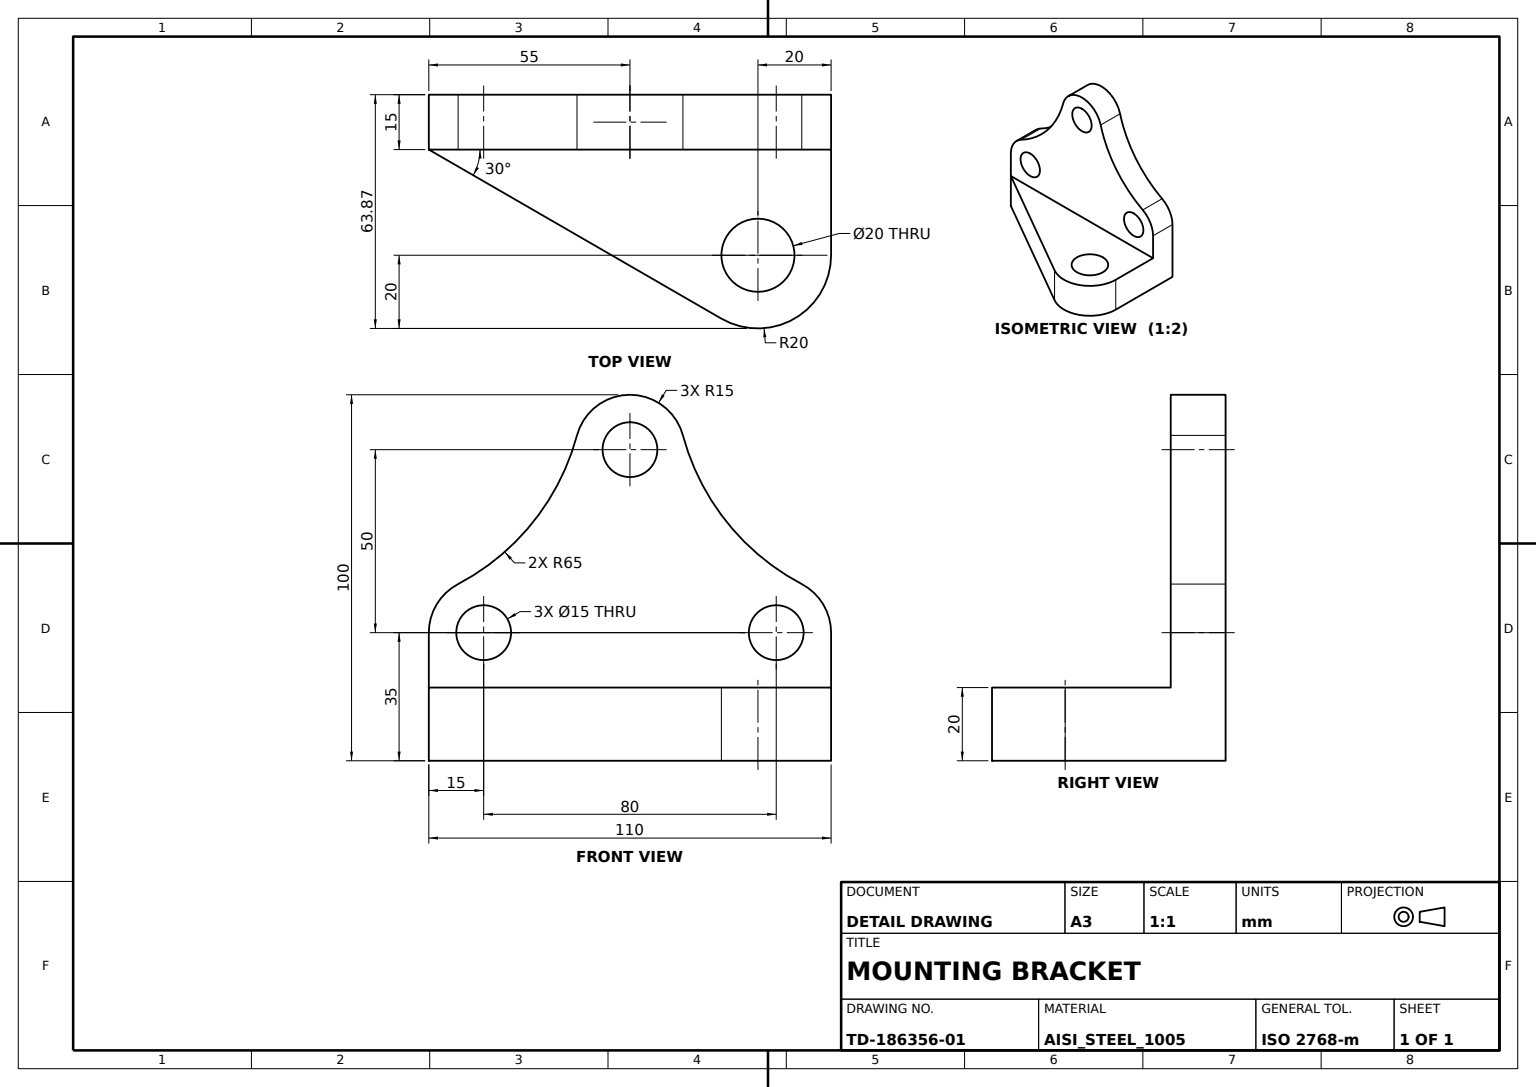
ISO-10303-21;
HEADER;
FILE_DESCRIPTION((''),'2;1');
FILE_NAME('','',(''),(''),'','','');
FILE_SCHEMA(('AUTOMOTIVE_DESIGN'));
ENDSEC;
DATA;
#1=APPLICATION_CONTEXT('');
#2=PRODUCT_CONTEXT('',#1,'mechanical');
#3=PRODUCT('','','',(#2));
#4=PRODUCT_DEFINITION_FORMATION('','',#3);
#5=PRODUCT_DEFINITION_CONTEXT('',#1,'design');
#6=PRODUCT_DEFINITION('','',#4,#5);
#7=PRODUCT_DEFINITION_SHAPE('','',#6);
#8=(LENGTH_UNIT()NAMED_UNIT(*)SI_UNIT(.MILLI.,.METRE.));
#9=(NAMED_UNIT(*)PLANE_ANGLE_UNIT()SI_UNIT($,.RADIAN.));
#10=(NAMED_UNIT(*)SI_UNIT($,.STERADIAN.)SOLID_ANGLE_UNIT());
#11=UNCERTAINTY_MEASURE_WITH_UNIT(LENGTH_MEASURE(0.005),#8,'distance_accuracy_value','');
#12=(GEOMETRIC_REPRESENTATION_CONTEXT(3)GLOBAL_UNCERTAINTY_ASSIGNED_CONTEXT((#11))GLOBAL_UNIT_ASSIGNED_CONTEXT((#8,#9,#10))REPRESENTATION_CONTEXT('',''));
#13=CARTESIAN_POINT('',(20.,0.,92.5));
#14=VERTEX_POINT('',#13);
#15=CARTESIAN_POINT('',(20.,0.,85.));
#16=DIRECTION('',(-1.,0.,0.));
#17=DIRECTION('',(0.,0.,1.));
#18=AXIS2_PLACEMENT_3D('',#15,#16,#17);
#19=CIRCLE('',#18,7.5);
#20=EDGE_CURVE('',#14,#14,#19,.T.);
#21=ORIENTED_EDGE('',*,*,#20,.T.);
#22=EDGE_LOOP('',(#21));
#23=FACE_BOUND('',#22,.T.);
#24=CARTESIAN_POINT('',(20.,40.,42.5));
#25=VERTEX_POINT('',#24);
#26=CARTESIAN_POINT('',(20.,40.,35.));
#27=AXIS2_PLACEMENT_3D('',#26,#16,#17);
#28=CIRCLE('',#27,7.5);
#29=EDGE_CURVE('',#25,#25,#28,.T.);
#30=ORIENTED_EDGE('',*,*,#29,.T.);
#31=EDGE_LOOP('',(#30));
#32=FACE_BOUND('',#31,.T.);
#33=CARTESIAN_POINT('',(20.,55.,20.));
#34=VERTEX_POINT('',#33);
#35=CARTESIAN_POINT('',(20.,55.,35.));
#36=VERTEX_POINT('',#35);
#37=CARTESIAN_POINT('',(20.,55.,0.));
#38=VECTOR('',#17,1000.);
#39=LINE('',#37,#38);
#40=EDGE_CURVE('',#34,#36,#39,.T.);
#41=ORIENTED_EDGE('',*,*,#40,.T.);
#42=CARTESIAN_POINT('',(20.,46.984173,48.274838));
#43=VERTEX_POINT('',#42);
#44=DIRECTION('',(1.,0.,0.));
#45=DIRECTION('',(0.,1.,0.));
#46=AXIS2_PLACEMENT_3D('',#26,#44,#45);
#47=CIRCLE('',#46,15.);
#48=EDGE_CURVE('',#36,#43,#47,.T.);
#49=ORIENTED_EDGE('',*,*,#48,.T.);
#50=CARTESIAN_POINT('',(20.,14.484173,88.899838));
#51=VERTEX_POINT('',#50);
#52=CARTESIAN_POINT('',(20.,77.248922,105.799137));
#53=DIRECTION('',(0.,-1.,0.));
#54=AXIS2_PLACEMENT_3D('',#52,#16,#53);
#55=CIRCLE('',#54,65.);
#56=EDGE_CURVE('',#43,#51,#55,.T.);
#57=ORIENTED_EDGE('',*,*,#56,.T.);
#58=CARTESIAN_POINT('',(20.,-14.484173,88.899838));
#59=VERTEX_POINT('',#58);
#60=AXIS2_PLACEMENT_3D('',#15,#44,#45);
#61=CIRCLE('',#60,15.);
#62=EDGE_CURVE('',#51,#59,#61,.T.);
#63=ORIENTED_EDGE('',*,*,#62,.T.);
#64=CARTESIAN_POINT('',(20.,-46.984173,48.274838));
#65=VERTEX_POINT('',#64);
#66=CARTESIAN_POINT('',(20.,-77.248922,105.799137));
#67=AXIS2_PLACEMENT_3D('',#66,#16,#45);
#68=CIRCLE('',#67,65.);
#69=EDGE_CURVE('',#59,#65,#68,.T.);
#70=ORIENTED_EDGE('',*,*,#69,.T.);
#71=CARTESIAN_POINT('',(20.,-55.,35.));
#72=VERTEX_POINT('',#71);
#73=CARTESIAN_POINT('',(20.,-40.,35.));
#74=AXIS2_PLACEMENT_3D('',#73,#44,#45);
#75=CIRCLE('',#74,15.);
#76=EDGE_CURVE('',#65,#72,#75,.T.);
#77=ORIENTED_EDGE('',*,*,#76,.T.);
#78=CARTESIAN_POINT('',(20.,-55.,20.));
#79=VERTEX_POINT('',#78);
#80=DIRECTION('',(0.,0.,-1.));
#81=VECTOR('',#80,1000.);
#82=LINE('',#71,#81);
#83=EDGE_CURVE('',#72,#79,#82,.T.);
#84=ORIENTED_EDGE('',*,*,#83,.T.);
#85=VECTOR('',#53,1000.);
#86=LINE('',#33,#85);
#87=EDGE_CURVE('',#34,#79,#86,.T.);
#88=ORIENTED_EDGE('',*,*,#87,.F.);
#89=EDGE_LOOP('',(#41,#49,#57,#63,#70,#77,#84,#88));
#90=FACE_BOUND('',#89,.T.);
#91=CARTESIAN_POINT('',(20.,-40.,42.5));
#92=VERTEX_POINT('',#91);
#93=AXIS2_PLACEMENT_3D('',#73,#16,#17);
#94=CIRCLE('',#93,7.5);
#95=EDGE_CURVE('',#92,#92,#94,.T.);
#96=ORIENTED_EDGE('',*,*,#95,.T.);
#97=EDGE_LOOP('',(#96));
#98=FACE_BOUND('',#97,.T.);
#99=AXIS2_PLACEMENT_3D('',#26,#44,#80);
#100=PLANE('',#99);
#101=ADVANCED_FACE('',(#23,#32,#90,#98),#100,.T.);
#102=ORIENTED_EDGE('',*,*,#95,.F.);
#103=EDGE_LOOP('',(#102));
#104=FACE_BOUND('',#103,.T.);
#105=CARTESIAN_POINT('',(5.,-40.,27.5));
#106=VERTEX_POINT('',#105);
#107=CARTESIAN_POINT('',(5.,-40.,35.));
#108=AXIS2_PLACEMENT_3D('',#107,#44,#80);
#109=CIRCLE('',#108,7.5);
#110=EDGE_CURVE('',#106,#106,#109,.T.);
#111=ORIENTED_EDGE('',*,*,#110,.F.);
#112=EDGE_LOOP('',(#111));
#113=FACE_BOUND('',#112,.T.);
#114=CYLINDRICAL_SURFACE('',#93,7.5);
#115=ADVANCED_FACE('',(#104,#113),#114,.F.);
#116=CARTESIAN_POINT('',(5.,40.,27.5));
#117=VERTEX_POINT('',#116);
#118=CARTESIAN_POINT('',(5.,40.,35.));
#119=AXIS2_PLACEMENT_3D('',#118,#44,#80);
#120=CIRCLE('',#119,7.5);
#121=EDGE_CURVE('',#117,#117,#120,.T.);
#122=ORIENTED_EDGE('',*,*,#121,.F.);
#123=EDGE_LOOP('',(#122));
#124=FACE_BOUND('',#123,.T.);
#125=ORIENTED_EDGE('',*,*,#29,.F.);
#126=EDGE_LOOP('',(#125));
#127=FACE_BOUND('',#126,.T.);
#128=CYLINDRICAL_SURFACE('',#27,7.5);
#129=ADVANCED_FACE('',(#124,#127),#128,.F.);
#130=CARTESIAN_POINT('',(66.188022,25.,20.));
#131=VERTEX_POINT('',#130);
#132=DIRECTION('',(0.5,0.866025404,0.));
#133=VECTOR('',#132,1000.);
#134=LINE('',#78,#133);
#135=EDGE_CURVE('',#79,#131,#134,.T.);
#136=ORIENTED_EDGE('',*,*,#135,.F.);
#137=CARTESIAN_POINT('',(20.,-55.,0.));
#138=VERTEX_POINT('',#137);
#139=LINE('',#78,#81);
#140=EDGE_CURVE('',#79,#138,#139,.T.);
#141=ORIENTED_EDGE('',*,*,#140,.T.);
#142=CARTESIAN_POINT('',(66.188022,25.,0.));
#143=VERTEX_POINT('',#142);
#144=LINE('',#137,#133);
#145=EDGE_CURVE('',#138,#143,#144,.T.);
#146=ORIENTED_EDGE('',*,*,#145,.T.);
#147=LINE('',#130,#81);
#148=EDGE_CURVE('',#131,#143,#147,.T.);
#149=ORIENTED_EDGE('',*,*,#148,.F.);
#150=EDGE_LOOP('',(#136,#141,#146,#149));
#151=FACE_BOUND('',#150,.T.);
#152=DIRECTION('',(-0.866025404,0.5,0.));
#153=DIRECTION('',(-0.5,-0.866025404,0.));
#154=AXIS2_PLACEMENT_3D('',#78,#152,#153);
#155=PLANE('',#154);
#156=ADVANCED_FACE('',(#151),#155,.F.);
#157=ORIENTED_EDGE('',*,*,#20,.F.);
#158=EDGE_LOOP('',(#157));
#159=FACE_BOUND('',#158,.T.);
#160=CARTESIAN_POINT('',(5.,0.,77.5));
#161=VERTEX_POINT('',#160);
#162=CARTESIAN_POINT('',(5.,0.,85.));
#163=AXIS2_PLACEMENT_3D('',#162,#44,#80);
#164=CIRCLE('',#163,7.5);
#165=EDGE_CURVE('',#161,#161,#164,.T.);
#166=ORIENTED_EDGE('',*,*,#165,.F.);
#167=EDGE_LOOP('',(#166));
#168=FACE_BOUND('',#167,.T.);
#169=CYLINDRICAL_SURFACE('',#18,7.5);
#170=ADVANCED_FACE('',(#159,#168),#169,.F.);
#171=ORIENTED_EDGE('',*,*,#165,.T.);
#172=EDGE_LOOP('',(#171));
#173=FACE_BOUND('',#172,.T.);
#174=CARTESIAN_POINT('',(5.,-55.,35.));
#175=VERTEX_POINT('',#174);
#176=CARTESIAN_POINT('',(5.,-55.,0.));
#177=VERTEX_POINT('',#176);
#178=LINE('',#174,#81);
#179=EDGE_CURVE('',#175,#177,#178,.T.);
#180=ORIENTED_EDGE('',*,*,#179,.F.);
#181=CARTESIAN_POINT('',(5.,-46.984173,48.274838));
#182=VERTEX_POINT('',#181);
#183=AXIS2_PLACEMENT_3D('',#107,#44,#45);
#184=CIRCLE('',#183,15.);
#185=EDGE_CURVE('',#182,#175,#184,.T.);
#186=ORIENTED_EDGE('',*,*,#185,.F.);
#187=CARTESIAN_POINT('',(5.,-14.484173,88.899838));
#188=VERTEX_POINT('',#187);
#189=CARTESIAN_POINT('',(5.,-77.248922,105.799137));
#190=AXIS2_PLACEMENT_3D('',#189,#16,#45);
#191=CIRCLE('',#190,65.);
#192=EDGE_CURVE('',#188,#182,#191,.T.);
#193=ORIENTED_EDGE('',*,*,#192,.F.);
#194=CARTESIAN_POINT('',(5.,14.484173,88.899838));
#195=VERTEX_POINT('',#194);
#196=AXIS2_PLACEMENT_3D('',#162,#44,#45);
#197=CIRCLE('',#196,15.);
#198=EDGE_CURVE('',#195,#188,#197,.T.);
#199=ORIENTED_EDGE('',*,*,#198,.F.);
#200=CARTESIAN_POINT('',(5.,46.984173,48.274838));
#201=VERTEX_POINT('',#200);
#202=CARTESIAN_POINT('',(5.,77.248922,105.799137));
#203=AXIS2_PLACEMENT_3D('',#202,#16,#53);
#204=CIRCLE('',#203,65.);
#205=EDGE_CURVE('',#201,#195,#204,.T.);
#206=ORIENTED_EDGE('',*,*,#205,.F.);
#207=CARTESIAN_POINT('',(5.,55.,35.));
#208=VERTEX_POINT('',#207);
#209=AXIS2_PLACEMENT_3D('',#118,#44,#45);
#210=CIRCLE('',#209,15.);
#211=EDGE_CURVE('',#208,#201,#210,.T.);
#212=ORIENTED_EDGE('',*,*,#211,.F.);
#213=CARTESIAN_POINT('',(5.,55.,0.));
#214=VERTEX_POINT('',#213);
#215=LINE('',#213,#38);
#216=EDGE_CURVE('',#214,#208,#215,.T.);
#217=ORIENTED_EDGE('',*,*,#216,.F.);
#218=VECTOR('',#45,1000.);
#219=LINE('',#176,#218);
#220=EDGE_CURVE('',#177,#214,#219,.T.);
#221=ORIENTED_EDGE('',*,*,#220,.F.);
#222=EDGE_LOOP('',(#180,#186,#193,#199,#206,#212,#217,#221));
#223=FACE_BOUND('',#222,.T.);
#224=ORIENTED_EDGE('',*,*,#121,.T.);
#225=EDGE_LOOP('',(#224));
#226=FACE_BOUND('',#225,.T.);
#227=ORIENTED_EDGE('',*,*,#110,.T.);
#228=EDGE_LOOP('',(#227));
#229=FACE_BOUND('',#228,.T.);
#230=PLANE('',#119);
#231=ADVANCED_FACE('',(#173,#223,#226,#229),#230,.F.);
#232=VECTOR('',#16,1000.);
#233=LINE('',#137,#232);
#234=EDGE_CURVE('',#138,#177,#233,.T.);
#235=ORIENTED_EDGE('',*,*,#234,.F.);
#236=ORIENTED_EDGE('',*,*,#140,.F.);
#237=ORIENTED_EDGE('',*,*,#83,.F.);
#238=LINE('',#71,#232);
#239=EDGE_CURVE('',#72,#175,#238,.T.);
#240=ORIENTED_EDGE('',*,*,#239,.T.);
#241=ORIENTED_EDGE('',*,*,#179,.T.);
#242=EDGE_LOOP('',(#235,#236,#237,#240,#241));
#243=FACE_BOUND('',#242,.T.);
#244=AXIS2_PLACEMENT_3D('',#71,#45,#17);
#245=PLANE('',#244);
#246=ADVANCED_FACE('',(#243),#245,.F.);
#247=ORIENTED_EDGE('',*,*,#62,.F.);
#248=LINE('',#50,#232);
#249=EDGE_CURVE('',#51,#195,#248,.T.);
#250=ORIENTED_EDGE('',*,*,#249,.T.);
#251=ORIENTED_EDGE('',*,*,#198,.T.);
#252=LINE('',#58,#232);
#253=EDGE_CURVE('',#59,#188,#252,.T.);
#254=ORIENTED_EDGE('',*,*,#253,.F.);
#255=EDGE_LOOP('',(#247,#250,#251,#254));
#256=FACE_BOUND('',#255,.T.);
#257=CYLINDRICAL_SURFACE('',#18,15.);
#258=ADVANCED_FACE('',(#256),#257,.T.);
#259=ORIENTED_EDGE('',*,*,#249,.F.);
#260=ORIENTED_EDGE('',*,*,#56,.F.);
#261=LINE('',#42,#232);
#262=EDGE_CURVE('',#43,#201,#261,.T.);
#263=ORIENTED_EDGE('',*,*,#262,.T.);
#264=ORIENTED_EDGE('',*,*,#205,.T.);
#265=EDGE_LOOP('',(#259,#260,#263,#264));
#266=FACE_BOUND('',#265,.T.);
#267=AXIS2_PLACEMENT_3D('',#52,#16,#17);
#268=CYLINDRICAL_SURFACE('',#267,65.);
#269=ADVANCED_FACE('',(#266),#268,.F.);
#270=CARTESIAN_POINT('',(38.867513,35.,20.));
#271=VERTEX_POINT('',#270);
#272=CARTESIAN_POINT('',(48.867513,35.,20.));
#273=AXIS2_PLACEMENT_3D('',#272,#80,#16);
#274=CIRCLE('',#273,10.);
#275=EDGE_CURVE('',#271,#271,#274,.T.);
#276=ORIENTED_EDGE('',*,*,#275,.F.);
#277=EDGE_LOOP('',(#276));
#278=FACE_BOUND('',#277,.T.);
#279=CARTESIAN_POINT('',(58.867513,35.,0.));
#280=VERTEX_POINT('',#279);
#281=CARTESIAN_POINT('',(48.867513,35.,0.));
#282=AXIS2_PLACEMENT_3D('',#281,#17,#44);
#283=CIRCLE('',#282,10.);
#284=EDGE_CURVE('',#280,#280,#283,.T.);
#285=ORIENTED_EDGE('',*,*,#284,.F.);
#286=EDGE_LOOP('',(#285));
#287=FACE_BOUND('',#286,.T.);
#288=CYLINDRICAL_SURFACE('',#273,10.);
#289=ADVANCED_FACE('',(#278,#287),#288,.F.);
#290=ORIENTED_EDGE('',*,*,#148,.T.);
#291=CARTESIAN_POINT('',(48.867513,55.,0.));
#292=VERTEX_POINT('',#291);
#293=CIRCLE('',#282,20.);
#294=EDGE_CURVE('',#143,#292,#293,.T.);
#295=ORIENTED_EDGE('',*,*,#294,.T.);
#296=CARTESIAN_POINT('',(48.867513,55.,20.));
#297=VERTEX_POINT('',#296);
#298=LINE('',#296,#81);
#299=EDGE_CURVE('',#297,#292,#298,.T.);
#300=ORIENTED_EDGE('',*,*,#299,.F.);
#301=AXIS2_PLACEMENT_3D('',#272,#17,#44);
#302=CIRCLE('',#301,20.);
#303=EDGE_CURVE('',#131,#297,#302,.T.);
#304=ORIENTED_EDGE('',*,*,#303,.F.);
#305=EDGE_LOOP('',(#290,#295,#300,#304));
#306=FACE_BOUND('',#305,.T.);
#307=CYLINDRICAL_SURFACE('',#273,20.);
#308=ADVANCED_FACE('',(#306),#307,.T.);
#309=ORIENTED_EDGE('',*,*,#87,.T.);
#310=ORIENTED_EDGE('',*,*,#135,.T.);
#311=ORIENTED_EDGE('',*,*,#303,.T.);
#312=LINE('',#296,#232);
#313=EDGE_CURVE('',#297,#34,#312,.T.);
#314=ORIENTED_EDGE('',*,*,#313,.T.);
#315=EDGE_LOOP('',(#309,#310,#311,#314));
#316=FACE_BOUND('',#315,.T.);
#317=ORIENTED_EDGE('',*,*,#275,.T.);
#318=EDGE_LOOP('',(#317));
#319=FACE_BOUND('',#318,.T.);
#320=PLANE('',#301);
#321=ADVANCED_FACE('',(#316,#319),#320,.T.);
#322=LINE('',#35,#232);
#323=EDGE_CURVE('',#36,#208,#322,.T.);
#324=ORIENTED_EDGE('',*,*,#323,.T.);
#325=ORIENTED_EDGE('',*,*,#211,.T.);
#326=ORIENTED_EDGE('',*,*,#262,.F.);
#327=ORIENTED_EDGE('',*,*,#48,.F.);
#328=EDGE_LOOP('',(#324,#325,#326,#327));
#329=FACE_BOUND('',#328,.T.);
#330=CYLINDRICAL_SURFACE('',#27,15.);
#331=ADVANCED_FACE('',(#329),#330,.T.);
#332=ORIENTED_EDGE('',*,*,#299,.T.);
#333=LINE('',#291,#232);
#334=EDGE_CURVE('',#292,#214,#333,.T.);
#335=ORIENTED_EDGE('',*,*,#334,.T.);
#336=ORIENTED_EDGE('',*,*,#216,.T.);
#337=ORIENTED_EDGE('',*,*,#323,.F.);
#338=ORIENTED_EDGE('',*,*,#40,.F.);
#339=ORIENTED_EDGE('',*,*,#313,.F.);
#340=EDGE_LOOP('',(#332,#335,#336,#337,#338,#339));
#341=FACE_BOUND('',#340,.T.);
#342=AXIS2_PLACEMENT_3D('',#296,#53,#80);
#343=PLANE('',#342);
#344=ADVANCED_FACE('',(#341),#343,.F.);
#345=ORIENTED_EDGE('',*,*,#284,.T.);
#346=EDGE_LOOP('',(#345));
#347=FACE_BOUND('',#346,.T.);
#348=ORIENTED_EDGE('',*,*,#294,.F.);
#349=ORIENTED_EDGE('',*,*,#145,.F.);
#350=ORIENTED_EDGE('',*,*,#234,.T.);
#351=ORIENTED_EDGE('',*,*,#220,.T.);
#352=ORIENTED_EDGE('',*,*,#334,.F.);
#353=EDGE_LOOP('',(#348,#349,#350,#351,#352));
#354=FACE_BOUND('',#353,.T.);
#355=PLANE('',#282);
#356=ADVANCED_FACE('',(#347,#354),#355,.F.);
#357=LINE('',#64,#232);
#358=EDGE_CURVE('',#65,#182,#357,.T.);
#359=ORIENTED_EDGE('',*,*,#358,.T.);
#360=ORIENTED_EDGE('',*,*,#185,.T.);
#361=ORIENTED_EDGE('',*,*,#239,.F.);
#362=ORIENTED_EDGE('',*,*,#76,.F.);
#363=EDGE_LOOP('',(#359,#360,#361,#362));
#364=FACE_BOUND('',#363,.T.);
#365=CYLINDRICAL_SURFACE('',#93,15.);
#366=ADVANCED_FACE('',(#364),#365,.T.);
#367=ORIENTED_EDGE('',*,*,#192,.T.);
#368=ORIENTED_EDGE('',*,*,#358,.F.);
#369=ORIENTED_EDGE('',*,*,#69,.F.);
#370=ORIENTED_EDGE('',*,*,#253,.T.);
#371=EDGE_LOOP('',(#367,#368,#369,#370));
#372=FACE_BOUND('',#371,.T.);
#373=AXIS2_PLACEMENT_3D('',#66,#16,#17);
#374=CYLINDRICAL_SURFACE('',#373,65.);
#375=ADVANCED_FACE('',(#372),#374,.F.);
#376=CLOSED_SHELL('',(#101,#115,#129,#156,#170,#231,#246,#258,#269,#289,#308,#321,#331,#344,#356,#366,#375));
#377=MANIFOLD_SOLID_BREP('',#376);
#378=ADVANCED_BREP_SHAPE_REPRESENTATION('',(#377),#12);
#379=SHAPE_DEFINITION_REPRESENTATION(#7,#378);
ENDSEC;
END-ISO-10303-21;
